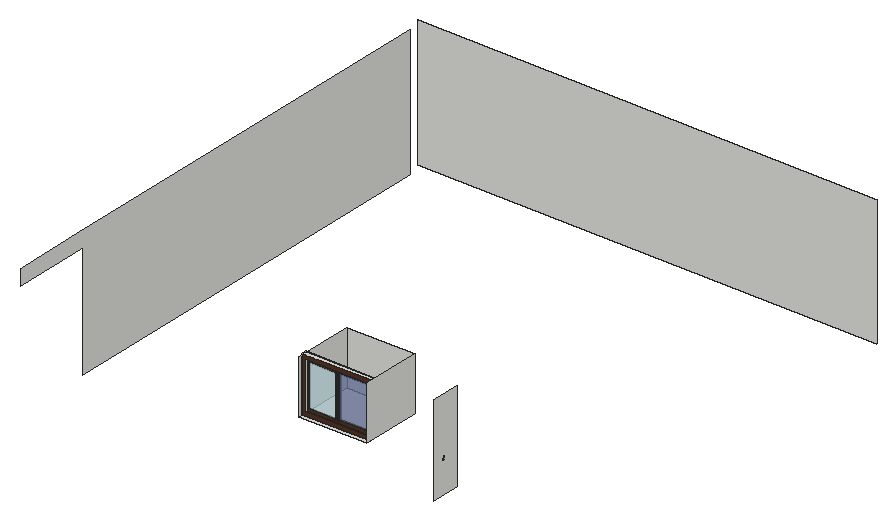
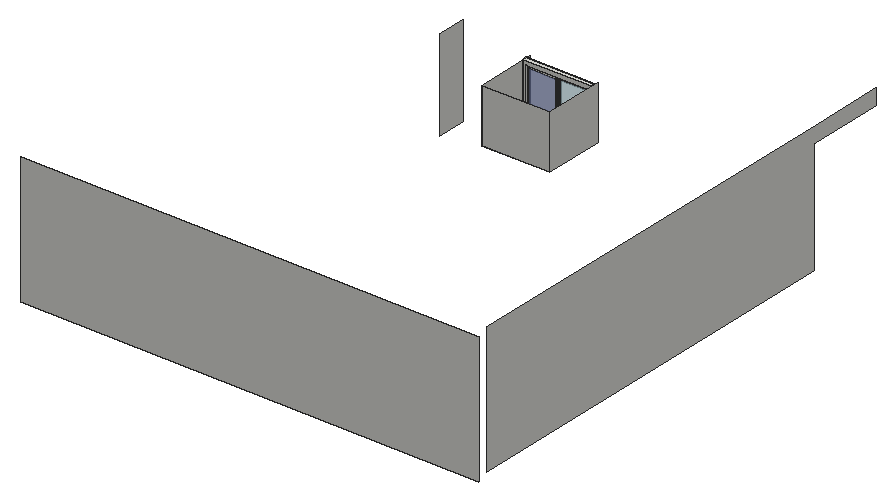
# SketchUp Ruby script. Lengths in inches.
U = 1.inch
M = Sketchup.active_model
def pt(a) = Geom::Point3d.new(a.map { |v| v * U })
def face(e, loops, mat)
  f = e.add_face(loops[0].map { |a| pt(a) })
  loops[1..].each { |l| e.add_face(l.map { |a| pt(a) }).erase! }
  f.material = f.back_material = mat if mat
  f
end
# faces: each face lists its corners as indices into pts; further lists are holes
def faces(e, pts, list, mat = nil) = list.each { |f| face(e, (f[0].is_a?(Array) ? f : [f]).map { |l| l.map { |i| pts[i] } }, mat) }
# xy, xz, yz: faces in a plane at the given z, y or x. An outline is a flat list of corners, or four numbers for a rectangle; further outlines are holes
def ring(l) = l.size == 4 ? [[l[0], l[1]], [l[2], l[1]], [l[2], l[3]], [l[0], l[3]]] : l.each_slice(2).to_a
def flat(e, list, mat, &to3) = list.each { |f| face(e, (f[0].is_a?(Array) ? f : [f]).map { |l| ring(l).map { |u, v| to3.(u, v) } }, mat) }
def xy(e, z, list, mat = nil) = flat(e, list, mat) { |x, y| [x, y, z] }
def xz(e, y, list, mat = nil) = flat(e, list, mat) { |x, z| [x, y, z] }
def yz(e, x, list, mat = nil) = flat(e, list, mat) { |y, z| [x, y, z] }
def lines(e, pts, list) = list.each { |a, b| e.add_line(pt(pts[a]), pt(pts[b])) }
# prism: a flat outline (further loops are holes) pulled along v
def prism(e, loops, v, mat = nil)
  f = face(e, loops, mat); d = Geom::Vector3d.new(v.map { |x| x * U })
  f.pushpull(f.normal.samedirection?(d) ? d.length : -d.length)
end
def box(e, o, s, mat = nil) = prism(e, [[o, [o[0] + s[0], o[1], o[2]], [o[0] + s[0], o[1] + s[1], o[2]], [o[0], o[1] + s[1], o[2]]]], [0, 0, s[2]], mat)
def at(x, y, z, deg = 0) = Geom::Transformation.translation(pt([x, y, z])) * Geom::Transformation.rotation(ORIGIN, Z_AXIS, deg.degrees)
def axes(o, x, y, z) = Geom::Transformation.new([*x, 0, *y, 0, *z, 0, *pt(o).to_a, 1])
def part(name) = M.definitions.add(name)
# library, detail: a bought-in or finely detailed component or shape, given as its bounding box
def library(name, o, s) = part(name).tap { |d| box(d.entities, o, s) }
def detail(e, o, s) = box(e.add_group.entities, o, s)
def put(e, d, t, mat = nil) = e.add_instance(d, t).tap { |i| i.material = mat if mat }
def group(e, t, mat = nil) = e.add_group.tap { |g| g.transformation = t; g.material = mat if mat }.entities
root = M.entities
M.materials.add("Material \#0").color = [86, 53, 35]
M.materials.add("Material \#1").color = [140, 140, 140]
M.materials.add("[Translucent_Glass_Safety]").color = [204, 235, 244]
M.materials["[Translucent_Glass_Safety]"].alpha = 0.5
M.materials.add("[Translucent_Glass_Sky_Reflection]").color = [125, 138, 183]
M.materials["[Translucent_Glass_Sky_Reflection]"].alpha = 0.52
c1 = part("Sliding window")
xy(c1.entities,0,[[0,0,4.33,55.51]])
xy(c1.entities,2.76,[[0,2.76,2,27.76],[3.15,2.76,4.33,27.76],[0,27.76,0.82,52.76],[0.82,27.76,2.36,52.76],[2.36,27.76,4.33,52.76]])
xy(c1.entities,4.72,[[2,4.72,2.4,26.38],[2.76,4.72,3.15,26.38],[0.82,29.13,1.22,50.79],[1.97,29.13,2.36,50.79]])
xy(c1.entities,36.61,[[2,4.72,2.4,26.38],[2.76,4.72,3.15,26.38],[0.82,29.13,1.22,50.79],[1.97,29.13,2.36,50.79]])
xy(c1.entities,38.58,[[0,2.76,2,27.76],[3.15,2.76,4.33,27.76],[0,27.76,0.82,52.76],[0.82,27.76,2.36,52.76],[2.36,27.76,4.33,52.76]])
xy(c1.entities,41.34,[[0,0,4.33,55.51]])
xz(c1.entities,0,[[0,0,4.33,41.34]])
xz(c1.entities,2.76,[[0,2.76,2,38.58],[3.15,2.76,4.33,38.58]])
xz(c1.entities,4.72,[[2,4.72,2.4,36.61],[2.76,4.72,3.15,36.61]])
xz(c1.entities,26.38,[[2,4.72,2.4,36.61],[2.76,4.72,3.15,36.61]])
xz(c1.entities,27.76,[[0.82,2.76,2,38.58],[2,2.76,2.36,38.58],[2.36,2.76,3.15,38.58]])
xz(c1.entities,29.13,[[0.82,4.72,1.22,36.61],[1.97,4.72,2.36,36.61]])
xz(c1.entities,50.79,[[0.82,4.72,1.22,36.61],[1.97,4.72,2.36,36.61]])
xz(c1.entities,52.76,[[0,2.76,0.82,38.58],[0.82,2.76,2.36,38.58],[2.36,2.76,4.33,38.58]])
xz(c1.entities,55.51,[[0,0,4.33,41.34]])
yz(c1.entities,0,[[[0,0,55.51,41.34],[2.76,2.76,52.76,38.58]]])
yz(c1.entities,0.82,[[[27.76,2.76,52.76,38.58],[29.13,4.72,50.79,36.61]]])
yz(c1.entities,1.22,[[29.13,4.72,50.79,36.61]],"[Translucent_Glass_Sky_Reflection]")
yz(c1.entities,1.97,[[29.13,4.72,50.79,36.61]],"[Translucent_Glass_Sky_Reflection]")
yz(c1.entities,2,[[[2.76,2.76,27.76,38.58],[4.72,4.72,26.38,36.61]]])
yz(c1.entities,2.36,[[[27.76,2.76,52.76,38.58],[29.13,4.72,50.79,36.61]]],"Material \#0")
yz(c1.entities,2.4,[[4.72,4.72,26.38,36.61]],"[Translucent_Glass_Safety]")
yz(c1.entities,2.76,[[4.72,4.72,26.38,36.61]],"[Translucent_Glass_Safety]")
yz(c1.entities,3.15,[[[2.76,2.76,27.76,38.58],[4.72,4.72,26.38,36.61]]],"Material \#0")
yz(c1.entities,4.33,[[[0,0,55.51,41.34],[2.76,2.76,52.76,38.58]]],"Material \#0")
xy(root,177.783,[[205.199,114.8125,268.449,169.8125]])
xz(root,116.631,[[338.056,187.336,338.056,187.348,337.928,187.348],[337.928,187.348,337.93,187.359,337.808,187.38],[337.928,187.348,338.056,187.348,337.93,187.359],[337.93,187.359,337.8125,187.391,337.808,187.38],[337.808,187.38,337.8125,187.391,337.698,187.431],
  [337.8125,187.391,337.704,187.441,337.698,187.431],[337.698,187.431,337.704,187.441,337.598,187.499],[337.704,187.441,337.606,187.508,337.598,187.499],[337.598,187.499,337.606,187.508,337.513,187.582],[337.606,187.508,337.522,187.59,337.513,187.582],
  [338.014,187.525,338.016,187.537,337.974,187.536],[338.014,187.525,338.056,187.533,338.016,187.537],[337.974,187.536,337.978,187.547,337.937,187.553],[337.974,187.536,338.016,187.537,337.978,187.547],[337.978,187.547,337.943,187.563,337.937,187.553],
  [337.513,187.582,337.522,187.59,337.446,187.673],[337.522,187.59,337.457,187.679,337.446,187.673],[337.875,187.603,337.885,187.611,337.852,187.635],[337.885,187.611,337.863,187.641,337.852,187.635],[337.852,187.635,337.863,187.641,337.835,187.671],
  [337.863,187.641,337.846,187.675,337.835,187.671],[337.835,187.671,337.846,187.675,337.824,187.71],[337.446,187.673,337.457,187.679,337.39,187.786],[337.846,187.675,337.836,187.712,337.824,187.71],[337.457,187.679,337.401,187.79,337.39,187.786],
  [337.824,187.71,337.836,187.712,337.82,187.747],[337.836,187.712,337.832,187.747,337.82,187.747],[337.82,187.747,337.832,187.747,337.824,187.792],[337.832,187.747,337.836,187.79,337.824,187.792],[337.39,187.786,337.401,187.79,337.357,187.903],
  [337.401,187.79,337.369,187.905,337.357,187.903],[337.836,187.79,337.835,187.831,337.824,187.792],[337.836,187.79,337.846,187.827,337.835,187.831],[337.846,187.827,337.852,187.867,337.835,187.831],[337.846,187.827,337.863,187.861,337.852,187.867],
  [337.863,187.861,337.875,187.899,337.852,187.867],[337.357,187.903,337.369,187.905,337.345,188.032],[337.369,187.905,337.357,188.032,337.345,188.032]],"Material \#1")
xz(root,116.666,[[338.056,189.714,337.935,189.77,337.988,189.729],[338.056,189.714,338.176,189.77,337.935,189.77],[338.056,189.714,337.988,189.729,338.02,189.718],[337.988,189.729,337.935,189.77,337.959,189.747],[338.176,189.77,337.782,190.362,337.896,190.174],
  [338.176,189.77,337.866,190.249,337.782,190.362],[338.176,189.77,337.903,190.212,337.866,190.249],[338.176,189.77,337.896,190.174,337.898,190.169],[338.176,189.77,337.898,190.169,337.9,190.163],[338.176,189.77,337.9,190.163,337.901,190.157],
  [337.935,189.77,337.901,190.151,337.906,189.829],[337.935,189.77,337.901,190.157,337.901,190.151],[337.935,189.77,338.176,189.77,337.901,190.157],[338.176,189.77,337.949,190.184,337.903,190.212],[337.935,189.77,337.906,189.829,337.917,189.798],
  [338.176,189.77,338,190.166,337.949,190.184],[337.906,189.829,337.901,190.151,337.901,189.864],[337.896,190.174,337.782,190.362,337.892,190.179],[337.892,190.179,337.782,190.362,337.888,190.184],[337.888,190.184,337.782,190.362,337.835,190.237],
  [337.888,190.184,337.835,190.237,337.882,190.188],[337.882,190.188,337.835,190.237,337.857,190.211],[337.835,190.237,337.782,190.362,337.8,190.295],[337.835,190.237,337.8,190.295,337.816,190.265],[337.866,190.249,337.837,190.293,337.782,190.362],
  [337.837,190.293,337.819,190.343,337.782,190.362],[337.8,190.295,337.782,190.362,337.789,190.327],[337.819,190.343,337.812,190.397,337.782,190.362],[337.782,190.362,337.787,190.459,337.78,190.397],[337.782,190.362,337.812,190.397,337.819,190.451],
  [337.782,190.362,337.819,190.451,337.84,190.565],[337.782,190.362,337.84,190.565,337.787,190.459],[337.819,190.451,337.837,190.501,337.84,190.565],[337.787,190.459,337.84,190.565,337.808,190.515],[337.837,190.501,337.866,190.545,337.84,190.565],
  [337.866,190.545,337.903,190.582,337.84,190.565],[337.84,190.565,337.903,190.582,337.949,190.61],[337.84,190.565,337.934,190.638,337.883,190.607],[337.84,190.565,337.949,190.61,338.056,190.666],[337.84,190.565,338.056,190.666,337.934,190.638],
  [337.949,190.61,338,190.628,338.056,190.666],[338,190.628,338.056,190.634,338.056,190.666],[337.934,190.638,338.056,190.666,337.993,190.659]],"Material \#1")
xz(root,116.676,[[338.056,190.186,338.056,190.194,338,190.193],[338.056,190.186,338.11,190.201,338.056,190.194],[338.056,190.186,338.112,190.193,338.11,190.201],[338,190.193,338.002,190.201,337.947,190.214],[338,190.193,338.056,190.194,338.002,190.201],
  [338.112,190.193,338.16,190.221,338.11,190.201],[338.112,190.193,338.164,190.214,338.16,190.221],[338.002,190.201,337.951,190.221,337.947,190.214],[337.947,190.214,337.951,190.221,337.902,190.248],[338.164,190.214,338.204,190.253,338.16,190.221],
  [338.164,190.214,338.209,190.248,338.204,190.253],[337.951,190.221,337.908,190.253,337.902,190.248],[337.902,190.248,337.908,190.253,337.868,190.291],[338.209,190.248,338.237,190.295,338.204,190.253],[338.209,190.248,338.244,190.291,338.237,190.295],
  [337.908,190.253,337.875,190.295,337.868,190.291],[337.868,190.291,337.875,190.295,337.846,190.342],[338.244,190.291,338.258,190.344,338.237,190.295],[338.244,190.291,338.266,190.342,338.258,190.344],[337.875,190.295,337.854,190.344,337.846,190.342],
  [337.846,190.342,337.854,190.344,337.839,190.397],[338.266,190.342,338.265,190.397,338.258,190.344],[338.266,190.342,338.273,190.397,338.265,190.397],[337.854,190.344,337.847,190.397,337.839,190.397],[337.839,190.397,337.847,190.397,337.846,190.452],
  [337.847,190.397,337.854,190.45,337.846,190.452],[338.265,190.397,338.273,190.397,338.258,190.45],[338.273,190.397,338.266,190.452,338.258,190.45],[337.854,190.45,337.868,190.503,337.846,190.452],[337.854,190.45,337.875,190.499,337.868,190.503],
  [338.258,190.45,338.266,190.452,338.237,190.499],[338.266,190.452,338.244,190.503,338.237,190.499],[337.875,190.499,337.902,190.546,337.868,190.503],[337.875,190.499,337.908,190.541,337.902,190.546],[338.237,190.499,338.244,190.503,338.204,190.541],
  [338.244,190.503,338.209,190.546,338.204,190.541],[337.908,190.541,337.947,190.58,337.902,190.546],[337.908,190.541,337.951,190.573,337.947,190.58],[338.204,190.541,338.209,190.546,338.16,190.573],[338.209,190.546,338.164,190.58,338.16,190.573],
  [337.951,190.573,338,190.601,337.947,190.58],[337.951,190.573,338.002,190.593,338,190.601],[338.16,190.573,338.164,190.58,338.11,190.593],[338.164,190.58,338.112,190.601,338.11,190.593],[338.002,190.593,338.056,190.608,338,190.601],
  [338.002,190.593,338.056,190.6,338.056,190.608],[338.11,190.593,338.112,190.601,338.056,190.6],[338.056,190.6,338.112,190.601,338.056,190.608]],"Material \#1")
xz(root,169.8125,[[205.199,177.783,268.449,227.533]])
xz(root,508.6875,[[0,141.9375,424.885,261.9375]])
yz(root,205.199,[[114.8125,177.783,169.8125,227.533]])
yz(root,268.449,[[114.8125,177.783,169.8125,227.533]])
yz(root,330.35,[[114.8125,151.779,141.3125,235.716]])
p = [[4.885,493.6875,141.9375],[4.885,493.6875,261.9375],[4.885,114.8125,261.9375],[4.884,42.5,261.9375],[4.885,42.5,247.422],[4.885,114.8125,247.422],
  [4.885,114.8125,141.9375]]
faces(root,p,[[0,1,2,3,4,5,6]])
put(root,c1,axes([205.2,122.83,177.78],[0,-1,0],[1.1394,0,0],[0,0,1.22464]))
